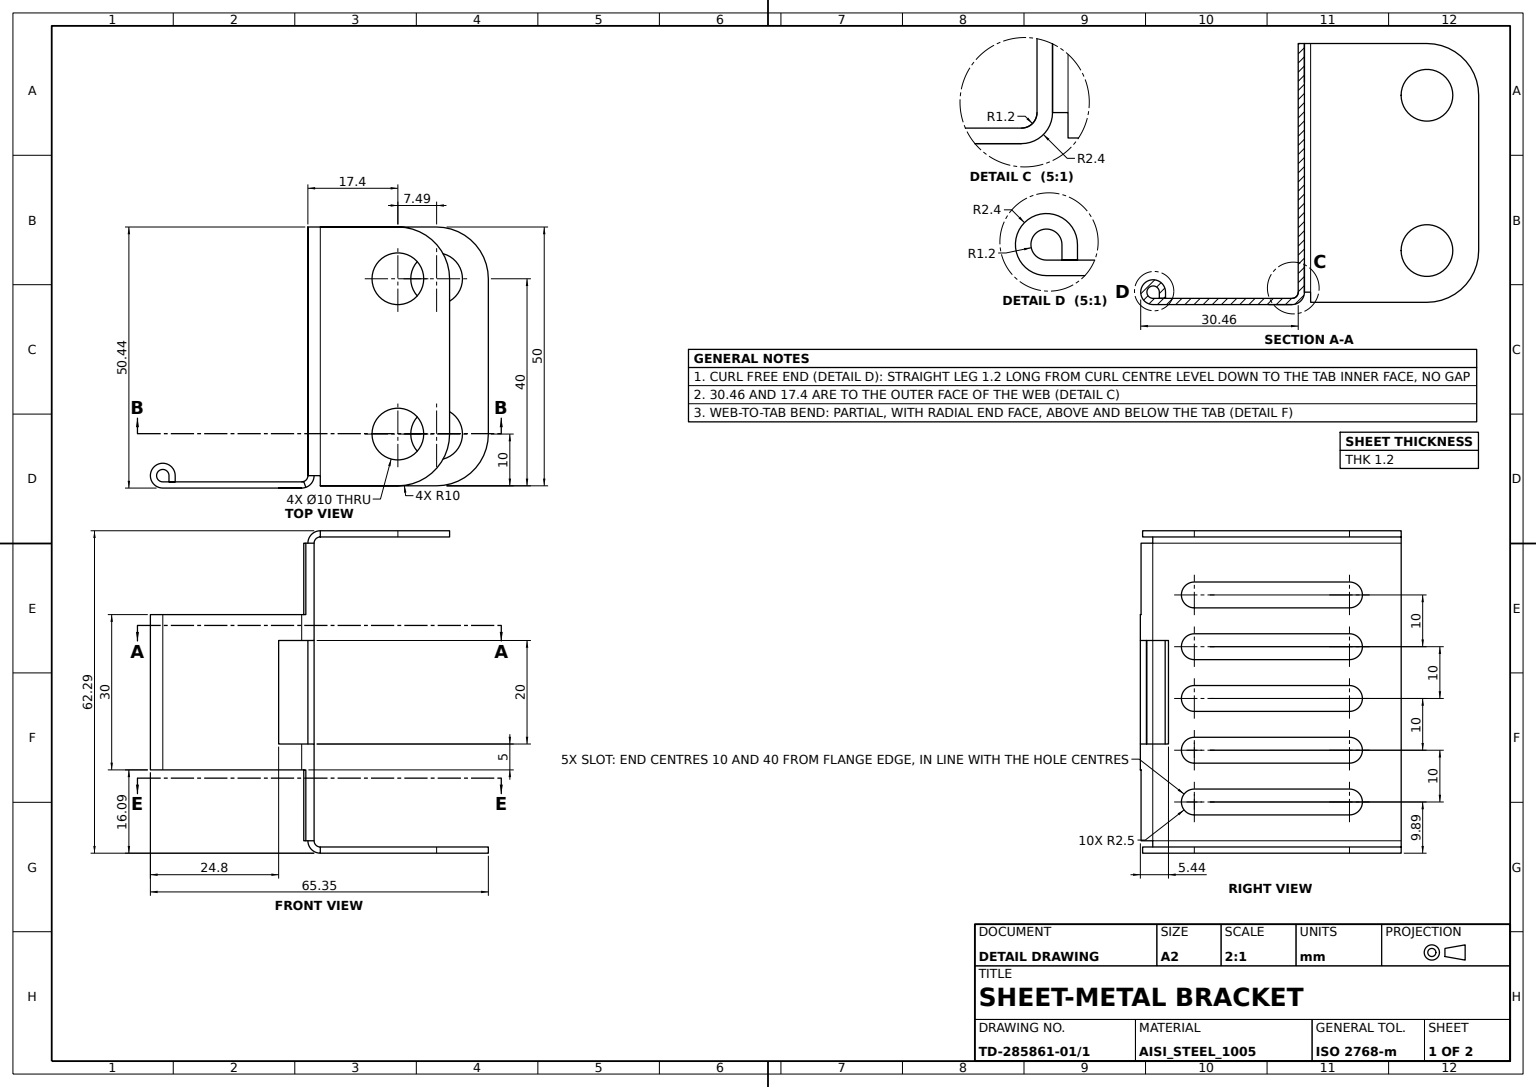
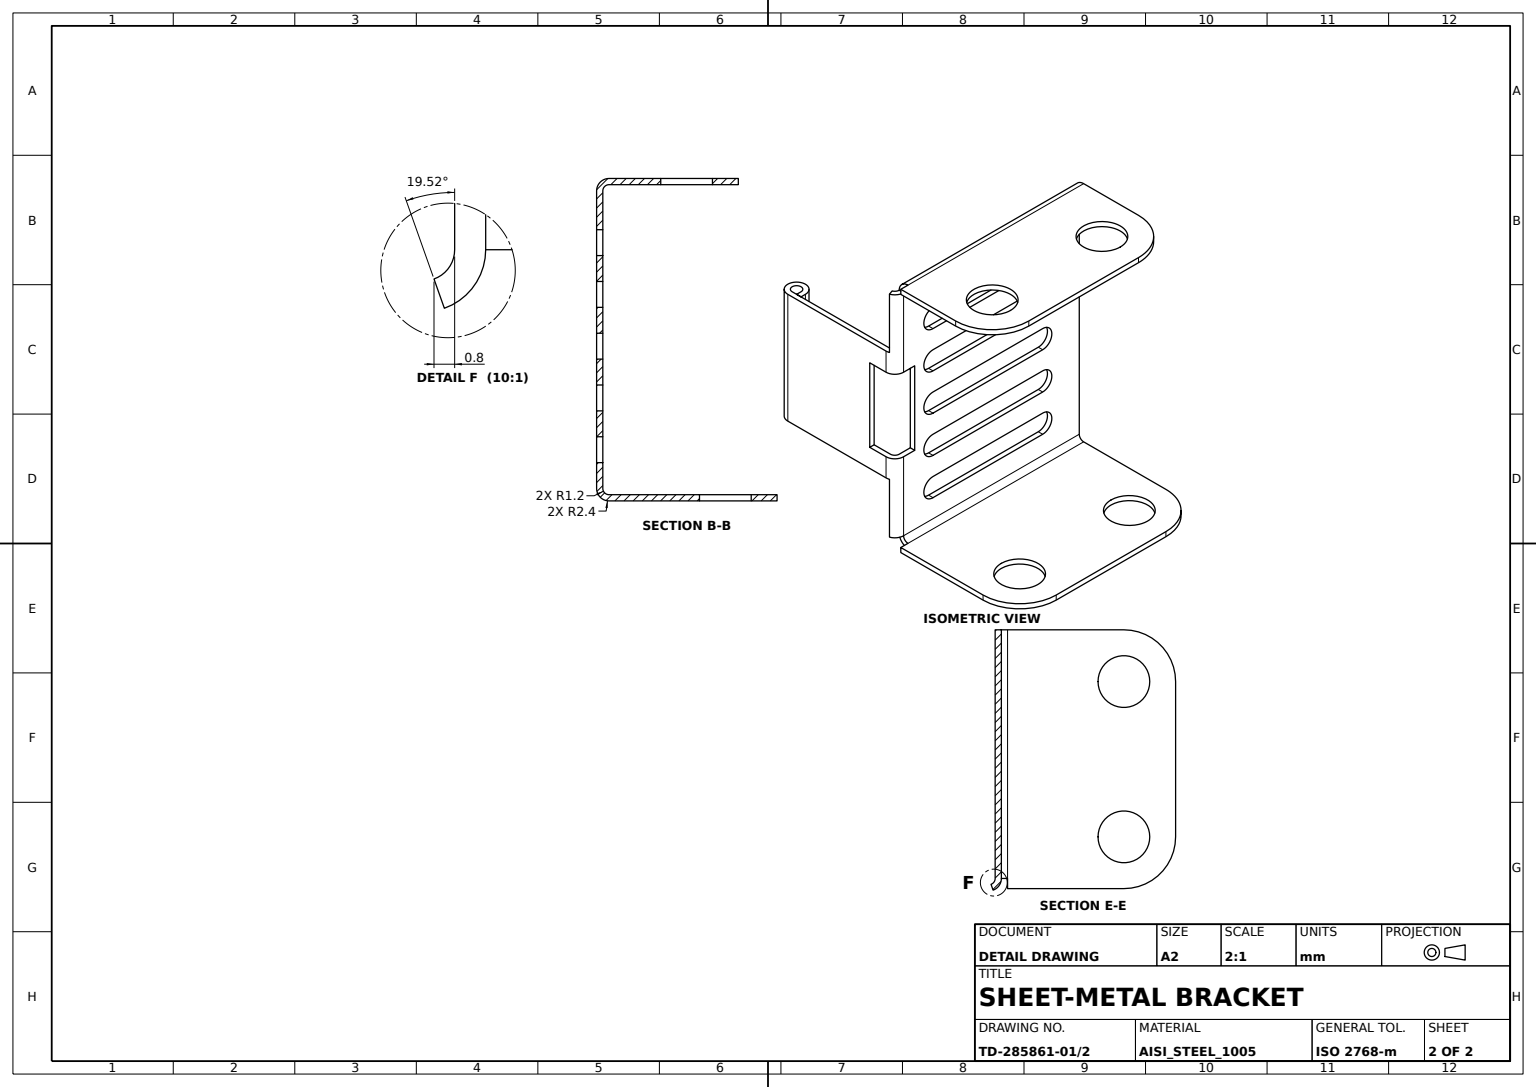
solid
v1 (33.8,14,-53.7)
v2 (32.6,14,-53.7)
e1 v1 v2 LINE
v3 (32.6,-16,-53.7)
e2 v2 v3 LINE
v4 (33.8,-16,-53.7)
e3 v4 v3 LINE
e4 v4 v1 LINE
face PLANE(AX(P(37.6,14,-53.7),D(0,0,-1),D(-1,0,0))) rev [e1 e2 -e3 e4]
v5 (32.6,-24.036746,-1.2)
v6 (33.8,-24.036746,-1.2)
e5 v5 v6 LINE
v7 (35,-24.036746,0)
e6 v6 v7 CIRCLE(AX(P(35,-24.036746,-1.2),D(0,-1,0),D(0,0,-1)),1.2) rev
v8 (35,-24.036746,1.2)
e7 v7 v8 LINE
e8 v8 v5 CIRCLE(AX(P(35,-24.036746,-1.2),D(0,1,0),D(0,0,1)),2.4) rev
face PLANE(AX(P(35,-24.036746,-1.2),D(0,1,0),D(0,0,1))) rev [e5 e6 e7 e8]
v9 (31.4,-25.236746,-45)
v10 (31.800962,-25.167776,-45)
e9 v9 v10 CIRCLE(AX(P(31.4,-24.036746,-45),D(0,0,-1),D(0,1,0)),1.2) rev
v11 (32.201923,-26.298806,-45)
e10 v10 v11 LINE
v12 (31.4,-26.436746,-45)
e11 v12 v11 CIRCLE(AX(P(31.4,-24.036746,-45),D(0,0,1),D(-1,0,0)),2.4)
v13 (4.543737,-26.436746,-45)
e12 v13 v12 LINE
v14 (6.943733,-24.032742,-45)
e13 v13 v14 CIRCLE(AX(P(4.543737,-24.036746,-45),D(0,0,-1),D(-1,0,0)),2.4)
v15 (6.945735,-25.232741,-45)
e14 v14 v15 LINE
v16 (5.745737,-25.234742,-45)
e15 v16 v15 LINE
v17 (5.743735,-24.034744,-45)
e16 v17 v16 LINE
v18 (4.543737,-25.236746,-45)
e17 v18 v17 CIRCLE(AX(P(4.543737,-24.036746,-45),D(0,0,-1),D(0,-1,0)),1.2)
e18 v18 v9 LINE
face PLANE(AX(P(2.143737,-26.436746,-45),D(0,0,1),D(0,-1,0))) rev [e9 e10 -e11 -e12 e13 e14 -e15 -e16 -e17 e18]
v19 (32.6,-16,-28.7)
v20 (32.6,14,-28.7)
e19 v19 v20 LINE
v21 (33.8,14,-28.7)
e20 v21 v20 LINE
v22 (33.8,-16,-28.7)
e21 v21 v22 LINE
e22 v22 v19 LINE
face PLANE(AX(P(37.6,-16,-28.7),D(0,0,1),D(1,0,0))) rev [e19 -e20 e21 e22]
v23 (57.493009,24,-59.893009)
v24 (35,24,-59.893009)
e23 v23 v24 LINE
v25 (57.493009,24,-61.093009)
e24 v25 v23 LINE
v26 (35,24,-61.093009)
e25 v25 v26 LINE
v27 (32.6,24,-58.693009)
e26 v26 v27 CIRCLE(AX(P(35,24,-58.693009),D(0,1,0),D(1,0,0)),2.4)
v28 (32.6,24,-1.2)
e27 v27 v28 LINE
v29 (35,24,1.2)
e28 v28 v29 CIRCLE(AX(P(35,24,-1.2),D(0,1,0),D(0,0,-1)),2.4)
v30 (50,24,1.2)
e29 v29 v30 LINE
v31 (50,24,0)
e30 v30 v31 LINE
v32 (35,24,0)
e31 v32 v31 LINE
v33 (33.8,24,-1.2)
e32 v33 v32 CIRCLE(AX(P(35,24,-1.2),D(0,-1,0),D(0,0,-1)),1.2) rev
v34 (33.8,24,-58.693009)
e33 v34 v33 LINE
e34 v24 v34 CIRCLE(AX(P(35,24,-58.693009),D(0,-1,0),D(0,0,1)),1.2) rev
face PLANE(AX(P(32.6,24,-83.693009),D(0,1,0),D(-1,0,0))) [-e23 -e24 e25 e26 e27 e28 e29 e30 -e31 -e32 -e33 -e34]
v35 (33.8,-16,-33.7)
v36 (32.6,-16,-33.7)
e35 v35 v36 LINE
e36 v36 v19 CIRCLE(AX(P(32.6,-16,-31.2),D(-1,0,0),D(0,0,1)),2.5)
e37 v22 v35 CIRCLE(AX(P(33.8,-16,-31.2),D(1,0,0),D(0,0,-1)),2.5)
face CYL(AX(P(37.6,-16,-31.2),D(-1,0,0),D(0,0,1)),2.5) rev [e35 e36 -e22 e37]
v37 (31.4,-25.236746,-15)
v38 (31.4,-25.236746,-20)
e38 v37 v38 LINE
v39 (31.800962,-25.167776,-15)
e39 v39 v37 CIRCLE(AX(P(31.4,-24.036746,-15),D(0,0,-1),D(0,1,0)),1.2)
v40 (31.800962,-25.167776,-1.2)
e40 v40 v39 LINE
e41 v40 v5 CIRCLE(AX(P(31.4,-24.036746,-1.2),D(0,0,-1),D(0,1,0)),1.2) rev
v41 (32.6,-24.036746,-20)
e42 v41 v5 LINE
e43 v38 v41 CIRCLE(AX(P(31.4,-24.036746,-20),D(0,0,-1),D(0,1,0)),1.2) rev
face CYL(AX(P(31.4,-24.036746,-40),D(0,0,-1),D(-1,0,0)),1.2) rev [-e38 -e39 -e40 e41 -e42 -e43]
v42 (67.493009,-16,-61.093009)
v43 (67.493009,-16,-59.893009)
e44 v42 v43 LINE
v44 (67.493009,14,-61.093009)
e45 v42 v44 LINE
v45 (67.493009,14,-59.893009)
e46 v44 v45 LINE
e47 v43 v45 LINE
face PLANE(AX(P(67.493009,-16,-61.093009),D(1,0,0),D(0,-1,0))) [-e44 e45 e46 -e47]
v46 (5.745737,-25.234742,-15)
e48 v46 v16 LINE
v47 (6.945735,-25.232741,-15)
e49 v47 v15 LINE
e50 v46 v47 LINE
face PLANE(AX(P(5.745737,-25.234742,-15),D(0.001668056,-0.999998609,0),D(0,0,-1))) [e48 e15 -e49 -e50]
v48 (35,-26,1.2)
v49 (35,-26,0)
e51 v48 v49 LINE
e52 v8 v48 LINE
e53 v49 v7 LINE
face PLANE(AX(P(35,24,1.2),D(1,0,0),D(0,0,-1))) rev [-e51 -e52 -e7 -e53]
v50 (33.8,-16,-23.7)
v51 (32.6,-16,-23.7)
e54 v50 v51 LINE
v52 (33.8,14,-23.7)
e55 v50 v52 LINE
v53 (32.6,14,-23.7)
e56 v52 v53 LINE
e57 v53 v51 LINE
face PLANE(AX(P(37.6,14,-23.7),D(0,0,-1),D(-1,0,0))) rev [-e54 e55 e56 e57]
v54 (57.493009,-26,-61.093009)
v55 (57.493009,-26,-59.893009)
e58 v54 v55 LINE
v56 (35,-26,-59.893009)
e59 v56 v55 LINE
v57 (35,-26,-61.093009)
e60 v57 v56 LINE
e61 v57 v54 LINE
face PLANE(AX(P(32.6,-26,16.306991),D(0,-1,0),D(1,0,0))) [e58 -e59 -e60 e61]
v58 (33.8,-24.036746,-58.693009)
v59 (35,-24.036746,-59.893009)
e62 v58 v59 CIRCLE(AX(P(35,-24.036746,-58.693009),D(0,1,0),D(0,0,1)),1.2) rev
e63 v24 v59 LINE
e64 v58 v34 LINE
face CYL(AX(P(35,24,-58.693009),D(0,-1,0),D(1,0,0)),1.2) rev [e62 -e63 e34 -e64]
v60 (50,-26,0)
e65 v60 v49 LINE
v61 (50,-26,1.2)
e66 v61 v60 LINE
e67 v61 v48 LINE
face PLANE(AX(P(32.6,-26,16.306991),D(0,-1,0),D(1,0,0))) [e51 -e65 -e66 e67]
v62 (26.943737,-26.436746,-40)
v63 (26.943737,-25.236746,-40)
e68 v62 v63 LINE
v64 (31.4,-26.436746,-40)
e69 v64 v62 LINE
v65 (33.8,-24.036746,-40)
e70 v65 v64 CIRCLE(AX(P(31.4,-24.036746,-40),D(0,0,-1),D(-1,0,0)),2.4)
v66 (33.8,-21,-40)
e71 v66 v65 LINE
v67 (32.6,-21,-40)
e72 v66 v67 LINE
v68 (32.6,-24.036746,-40)
e73 v68 v67 LINE
v69 (31.4,-25.236746,-40)
e74 v68 v69 CIRCLE(AX(P(31.4,-24.036746,-40),D(0,0,-1),D(0,1,0)),1.2)
e75 v63 v69 LINE
face PLANE(AX(P(37.6,-31,-40),D(0,0,1),D(1,0,0))) [-e68 -e69 -e70 -e71 e72 -e73 e74 -e75]
e76 v5 v28 LINE
e77 v29 v8 LINE
face CYL(AX(P(35,24,-1.2),D(0,-1,0),D(0,0,-1)),2.4) [-e28 -e76 -e8 -e77]
v70 (35,-24.036746,-61.093009)
e78 v70 v26 LINE
v71 (32.6,-24.036746,-58.693009)
e79 v70 v71 CIRCLE(AX(P(35,-24.036746,-58.693009),D(0,-1,0),D(0,0,-1)),2.4) rev
e80 v27 v71 LINE
face CYL(AX(P(35,24,-58.693009),D(0,-1,0),D(1,0,0)),2.4) [-e78 e79 -e80 -e26]
v72 (60,-16,1.2)
v73 (60,-16,0)
e81 v72 v73 LINE
e82 v72 v61 CIRCLE(AX(P(50,-16,1.2),D(0,0,-1),D(1,0,0)),10)
e83 v73 v60 CIRCLE(AX(P(50,-16,0),D(0,0,-1),D(1,0,0)),10)
face CYL(AX(P(50,-16,1.2),D(0,0,-1),D(-1,0,0)),10) [-e81 e82 e66 -e83]
v74 (26.943737,-25.236746,-20)
e84 v74 v63 LINE
e85 v69 v9 LINE
v75 (4.543737,-25.236746,-15)
e86 v75 v18 LINE
e87 v37 v75 LINE
e88 v38 v74 LINE
face PLANE(AX(P(41.943737,-25.236746,-83.693009),D(0,-1,0),D(0,0,-1))) rev [e84 e75 e85 -e18 -e86 -e87 e38 e88]
v76 (33.8,14,-33.7)
e89 v35 v76 LINE
e90 v76 v21 CIRCLE(AX(P(33.8,14,-31.2),D(1,0,0),D(0,0,-1)),2.5)
v77 (33.8,-16,-48.7)
e91 v77 v4 CIRCLE(AX(P(33.8,-16,-51.2),D(1,0,0),D(0,0,-1)),2.5)
v78 (33.8,14,-48.7)
e92 v78 v77 LINE
e93 v1 v78 CIRCLE(AX(P(33.8,14,-51.2),D(1,0,0),D(0,0,-1)),2.5)
v79 (33.8,-16,-18.7)
e94 v79 v50 CIRCLE(AX(P(33.8,-16,-21.2),D(1,0,0),D(0,0,-1)),2.5)
v80 (33.8,14,-18.7)
e95 v80 v79 LINE
e96 v52 v80 CIRCLE(AX(P(33.8,14,-21.2),D(1,0,0),D(0,0,-1)),2.5)
e97 v58 v65 LINE
e98 v33 v6 LINE
v81 (33.8,-24.036746,-20)
e99 v81 v6 LINE
v82 (33.8,-21,-20)
e100 v81 v82 LINE
e101 v82 v66 LINE
v83 (33.8,-16,-8.7)
v84 (33.8,-16,-13.7)
e102 v83 v84 CIRCLE(AX(P(33.8,-16,-11.2),D(1,0,0),D(0,0,-1)),2.5)
v85 (33.8,14,-8.7)
e103 v85 v83 LINE
v86 (33.8,14,-13.7)
e104 v86 v85 CIRCLE(AX(P(33.8,14,-11.2),D(1,0,0),D(0,0,-1)),2.5)
e105 v84 v86 LINE
v87 (33.8,-16,-38.7)
v88 (33.8,-16,-43.7)
e106 v87 v88 CIRCLE(AX(P(33.8,-16,-41.2),D(1,0,0),D(0,0,-1)),2.5)
v89 (33.8,14,-38.7)
e107 v89 v87 LINE
v90 (33.8,14,-43.7)
e108 v90 v89 CIRCLE(AX(P(33.8,14,-41.2),D(1,0,0),D(0,0,-1)),2.5)
e109 v88 v90 LINE
face PLANE(AX(P(33.8,-16,-83.693009),D(1,0,0),D(0,0,-1))) [-e89 -e37 -e21 -e90] [-e4 -e91 -e92 -e93] [-e55 -e94 -e95 -e96] [e71 -e97 e64 e33 e98 -e99 e100 e101] [-e102 -e103 -e104 -e105] [-e106 -e107 -e108 -e109]
v91 (32.6,-16,-43.7)
v92 (32.6,-16,-38.7)
e110 v91 v92 CIRCLE(AX(P(32.6,-16,-41.2),D(-1,0,0),D(0,0,1)),2.5)
e111 v87 v92 LINE
e112 v88 v91 LINE
face CYL(AX(P(37.6,-16,-41.2),D(-1,0,0),D(0,0,1)),2.5) rev [e110 -e111 e106 e112]
v93 (55,14,1.2)
e113 v93 v93 CIRCLE(AX(P(50,14,1.2),D(0,0,1),D(1,0,0)),5)
v94 (55,14,0)
e114 v94 v94 CIRCLE(AX(P(50,14,0),D(0,0,1),D(1,0,0)),5)
face CYL(AX(P(50,14,1.2),D(0,0,-1),D(-1,0,0)),5) rev [e113] [-e114]
v95 (32.6,14,-13.7)
e115 v86 v95 LINE
v96 (32.6,14,-8.7)
e116 v85 v96 LINE
e117 v96 v95 CIRCLE(AX(P(32.6,14,-11.2),D(-1,0,0),D(0,0,1)),2.5)
face CYL(AX(P(37.6,14,-11.2),D(-1,0,0),D(0,0,1)),2.5) rev [-e115 e104 e116 e117]
v97 (32.6,14,-33.7)
e118 v97 v36 LINE
e119 v20 v97 CIRCLE(AX(P(32.6,14,-31.2),D(-1,0,0),D(0,0,1)),2.5)
e120 v71 v68 LINE
v98 (32.6,-21,-20)
e121 v67 v98 LINE
e122 v98 v41 LINE
v99 (32.6,14,-18.7)
e123 v99 v53 CIRCLE(AX(P(32.6,14,-21.2),D(-1,0,0),D(0,0,1)),2.5)
v100 (32.6,-16,-18.7)
e124 v100 v99 LINE
e125 v51 v100 CIRCLE(AX(P(32.6,-16,-21.2),D(-1,0,0),D(0,0,1)),2.5)
v101 (32.6,14,-43.7)
e126 v101 v91 LINE
v102 (32.6,14,-38.7)
e127 v102 v101 CIRCLE(AX(P(32.6,14,-41.2),D(-1,0,0),D(0,0,1)),2.5)
e128 v92 v102 LINE
v103 (32.6,-16,-48.7)
e129 v3 v103 CIRCLE(AX(P(32.6,-16,-51.2),D(-1,0,0),D(0,0,1)),2.5)
v104 (32.6,14,-48.7)
e130 v104 v2 CIRCLE(AX(P(32.6,14,-51.2),D(-1,0,0),D(0,0,1)),2.5)
e131 v103 v104 LINE
v105 (32.6,-16,-8.7)
e132 v105 v96 LINE
v106 (32.6,-16,-13.7)
e133 v106 v105 CIRCLE(AX(P(32.6,-16,-11.2),D(-1,0,0),D(0,0,1)),2.5)
e134 v95 v106 LINE
face PLANE(AX(P(32.6,-16,-83.693009),D(1,0,0),D(0,0,-1))) rev [-e19 -e36 -e118 -e119] [e42 e76 -e27 e80 e120 e73 e121 e122] [-e123 -e124 -e125 -e57] [-e126 -e127 -e128 -e110] [-e129 -e2 -e130 -e131] [-e117 -e132 -e133 -e134]
e135 v83 v105 LINE
face PLANE(AX(P(37.6,-16,-8.7),D(0,0,1),D(1,0,0))) rev [e135 e132 -e116 e103]
v107 (31.4,-26.436746,-20)
e136 v107 v81 CIRCLE(AX(P(31.4,-24.036746,-20),D(0,0,1),D(-1,0,0)),2.4)
v108 (32.201923,-26.298806,-1.2)
e137 v108 v6 CIRCLE(AX(P(31.4,-24.036746,-1.2),D(0,0,1),D(-1,0,0)),2.4)
v109 (32.201923,-26.298806,-15)
e138 v108 v109 LINE
v110 (31.4,-26.436746,-15)
e139 v109 v110 CIRCLE(AX(P(31.4,-24.036746,-15),D(0,0,-1),D(-1,0,0)),2.4)
e140 v110 v107 LINE
face CYL(AX(P(31.4,-24.036746,-40),D(0,0,-1),D(-1,0,0)),2.4) [e136 e99 -e137 e138 e139 e140]
v111 (31.800962,-25.167776,-58.693009)
v112 (32.201923,-26.298806,-58.693009)
e141 v111 v112 LINE
e142 v111 v71 CIRCLE(AX(P(31.4,-24.036746,-58.693009),D(0,0,-1),D(0,1,0)),1.2) rev
e143 v71 v58 LINE
e144 v112 v58 CIRCLE(AX(P(31.4,-24.036746,-58.693009),D(0,0,1),D(-1,0,0)),2.4)
face PLANE(AX(P(31.4,-24.036746,-58.693009),D(0,0,-1),D(0,1,0))) [-e141 e142 e143 -e144]
e145 v76 v97 LINE
face PLANE(AX(P(37.6,14,-33.7),D(0,0,-1),D(-1,0,0))) rev [-e35 e89 e145 e118]
v113 (6.943733,-24.032742,-15)
e146 v113 v47 LINE
e147 v113 v14 LINE
face PLANE(AX(P(6.943733,-24.032742,-15),D(0.999998609,0.001668056,0),D(-0.001668056,0.999998609,0))) [e146 e49 -e14 -e147]
e148 v45 v23 CIRCLE(AX(P(57.493009,14,-59.893009),D(0,0,1),D(-1,0,0)),10)
e149 v44 v25 CIRCLE(AX(P(57.493009,14,-61.093009),D(0,0,1),D(-1,0,0)),10)
face CYL(AX(P(57.493009,14,-61.093009),D(0,0,1),D(1,0,0)),10) [-e148 -e46 e149 e24]
e150 v55 v43 CIRCLE(AX(P(57.493009,-16,-59.893009),D(0,0,1),D(-1,0,0)),10)
e151 v54 v42 CIRCLE(AX(P(57.493009,-16,-61.093009),D(0,0,1),D(-1,0,0)),10)
face CYL(AX(P(57.493009,-16,-61.093009),D(0,0,1),D(1,0,0)),10) [e44 -e150 -e58 e151]
v114 (55,-16,1.2)
e152 v114 v114 CIRCLE(AX(P(50,-16,1.2),D(0,0,1),D(1,0,0)),5)
v115 (55,-16,0)
e153 v115 v115 CIRCLE(AX(P(50,-16,0),D(0,0,1),D(1,0,0)),5)
face CYL(AX(P(50,-16,1.2),D(0,0,-1),D(-1,0,0)),5) rev [e152] [-e153]
v116 (4.543737,-26.436746,-15)
e154 v116 v13 LINE
e155 v116 v113 CIRCLE(AX(P(4.543737,-24.036746,-15),D(0,0,-1),D(-1,0,0)),2.4)
face CYL(AX(P(4.543737,-24.036746,-15),D(0,0,-1),D(-1,0,0)),2.4) [e147 -e13 -e154 e155]
e156 v89 v102 LINE
face PLANE(AX(P(37.6,-16,-38.7),D(0,0,1),D(1,0,0))) rev [e128 -e156 e107 e111]
e157 v80 v99 LINE
face CYL(AX(P(37.6,14,-21.2),D(-1,0,0),D(0,0,1)),2.5) rev [e96 e157 e123 -e56]
v117 (52.493009,-16,-59.893009)
e158 v117 v117 CIRCLE(AX(P(57.493009,-16,-59.893009),D(0,0,-1),D(-1,0,0)),5)
v118 (52.493009,-16,-61.093009)
e159 v118 v118 CIRCLE(AX(P(57.493009,-16,-61.093009),D(0,0,-1),D(-1,0,0)),5)
face CYL(AX(P(57.493009,-16,-61.093009),D(0,0,1),D(1,0,0)),5) rev [-e158] [e159]
e160 v79 v100 LINE
face PLANE(AX(P(37.6,-16,-18.7),D(0,0,1),D(1,0,0))) rev [e160 e124 -e157 e95]
e161 v82 v98 LINE
v119 (26.943737,-26.436746,-20)
e162 v119 v107 LINE
e163 v119 v74 LINE
face PLANE(AX(P(37.6,-21,-20),D(0,0,-1),D(-1,0,0))) [e43 -e122 -e161 -e100 -e136 -e162 e163 -e88]
e164 v64 v12 LINE
e165 v11 v112 LINE
face CYL(AX(P(31.4,-24.036746,-40),D(0,0,-1),D(-1,0,0)),2.4) [e164 e11 e165 e144 e97 e70]
e166 v77 v103 LINE
face CYL(AX(P(37.6,-16,-51.2),D(-1,0,0),D(0,0,1)),2.5) rev [e3 e129 -e166 e91]
face CYL(AX(P(37.6,-16,-21.2),D(-1,0,0),D(0,0,1)),2.5) rev [e94 e54 e125 -e160]
v120 (60,14,1.2)
e167 v120 v72 LINE
e168 v30 v120 CIRCLE(AX(P(50,14,1.2),D(0,0,-1),D(1,0,0)),10)
face PLANE(AX(P(-50,-16,1.2),D(0,0,-1),D(-1,0,0))) rev [-e113] [e77 e52 -e67 -e82 -e167 -e168 -e29] [-e152]
e169 v78 v104 LINE
face CYL(AX(P(37.6,14,-51.2),D(-1,0,0),D(0,0,1)),2.5) rev [e93 e169 e130 -e1]
e170 v56 v59 LINE
v121 (52.493009,14,-59.893009)
e171 v121 v121 CIRCLE(AX(P(57.493009,14,-59.893009),D(0,0,-1),D(-1,0,0)),5)
face PLANE(AX(P(57.493009,-16,-59.893009),D(0,0,1),D(1,0,0))) [e23 e63 -e170 e59 e150 e47 e148] [e171] [e158]
v122 (60,14,0)
e172 v120 v122 LINE
e173 v31 v122 CIRCLE(AX(P(50,14,0),D(0,0,-1),D(1,0,0)),10)
face CYL(AX(P(50,14,1.2),D(0,0,-1),D(-1,0,0)),10) [-e30 e168 e172 -e173]
e174 v57 v70 LINE
v123 (52.493009,14,-61.093009)
e175 v123 v123 CIRCLE(AX(P(57.493009,14,-61.093009),D(0,0,-1),D(-1,0,0)),5)
face PLANE(AX(P(57.493009,-16,-61.093009),D(0,0,1),D(1,0,0))) rev [-e61 e174 e78 -e25 -e149 -e45 -e151] [-e175] [-e159]
face PLANE(AX(P(37.6,-16,-48.7),D(0,0,1),D(1,0,0))) rev [-e169 e92 e166 e131]
e176 v62 v119 LINE
face PLANE(AX(P(26.943737,-30.236746,-20),D(1,0,0),D(0,0,1))) [-e84 -e163 -e176 e68]
v124 (5.743735,-24.034744,-15)
e177 v124 v17 LINE
e178 v75 v124 CIRCLE(AX(P(4.543737,-24.036746,-15),D(0,0,-1),D(0,-1,0)),1.2)
face CYL(AX(P(4.543737,-24.036746,-15),D(0,0,-1),D(-1,0,0)),1.2) rev [-e177 -e178 e86 e17]
e179 v122 v73 LINE
face PLANE(AX(P(60,14,1.2),D(1,0,0),D(0,1,0))) [e81 -e179 -e172 e167]
e180 v90 v101 LINE
face PLANE(AX(P(37.6,14,-43.7),D(0,0,-1),D(-1,0,0))) rev [e180 e126 -e112 e109]
e181 v7 v32 LINE
face CYL(AX(P(35,24,-1.2),D(0,-1,0),D(0,0,-1)),1.2) rev [-e6 -e98 e32 -e181]
e182 v110 v116 LINE
face PLANE(AX(P(41.943737,-26.436746,-83.693009),D(0,-1,0),D(0,0,-1))) [-e164 e69 e176 e162 -e140 e182 e154 e12]
face CYL(AX(P(37.6,14,-41.2),D(-1,0,0),D(0,0,1)),2.5) rev [e127 -e180 e108 e156]
face CYL(AX(P(57.493009,14,-61.093009),D(0,0,1),D(1,0,0)),5) rev [-e171] [e175]
e183 v39 v109 LINE
e184 v40 v108 LINE
face PLANE(AX(P(32.201923,-26.298806,-8.1),D(-0.942525313,-0.334134756,0),D(0,0,-1))) [e40 e183 -e138 -e184]
e185 v84 v106 LINE
face CYL(AX(P(37.6,-16,-11.2),D(-1,0,0),D(0,0,1)),2.5) rev [e133 -e135 e102 e185]
e186 v59 v70 LINE
face PLANE(AX(P(35,-24.036746,-58.693009),D(0,-1,0),D(0,0,-1))) [-e143 -e79 -e186 -e62]
e187 v10 v111 LINE
face PLANE(AX(P(32.201923,-26.298806,-51.846505),D(-0.942525313,-0.334134756,0),D(0,0,-1))) [e187 e141 -e165 -e10]
face CYL(AX(P(37.6,14,-31.2),D(-1,0,0),D(0,0,1)),2.5) rev [e20 e119 -e145 e90]
face PLANE(AX(P(-50,-16,0),D(0,0,-1),D(-1,0,0))) [e153] [e114] [e179 e83 e65 e53 e181 e31 e173]
e188 v124 v46 LINE
face PLANE(AX(P(5.743735,-24.034744,-15),D(0.999998609,0.001668056,0),D(-0.001668056,0.999998609,0))) rev [e177 e16 -e48 -e188]
face PLANE(AX(P(31.4,-24.036746,-1.2),D(0,0,-1),D(0,1,0))) rev [e184 e137 -e5 -e41]
face CYL(AX(P(31.4,-24.036746,-40),D(0,0,-1),D(-1,0,0)),1.2) rev [-e142 -e187 -e9 -e85 -e74 -e120]
face PLANE(AX(P(37.6,-21,-40),D(0,-1,0),D(0,0,-1))) [-e101 e161 -e121 -e72]
face PLANE(AX(P(37.6,14,-13.7),D(0,0,-1),D(-1,0,0))) rev [e134 -e185 e105 e115]
face PLANE(AX(P(31.943737,-26.436746,-15),D(0,0,-1),D(0,1,0))) rev [-e155 -e182 -e139 -e183 e39 e87 e178 e188 e50 -e146]
face PLANE(AX(P(35,24,-61.093009),D(1,0,0),D(0,1,0))) rev [e170 e186 -e174 e60]
